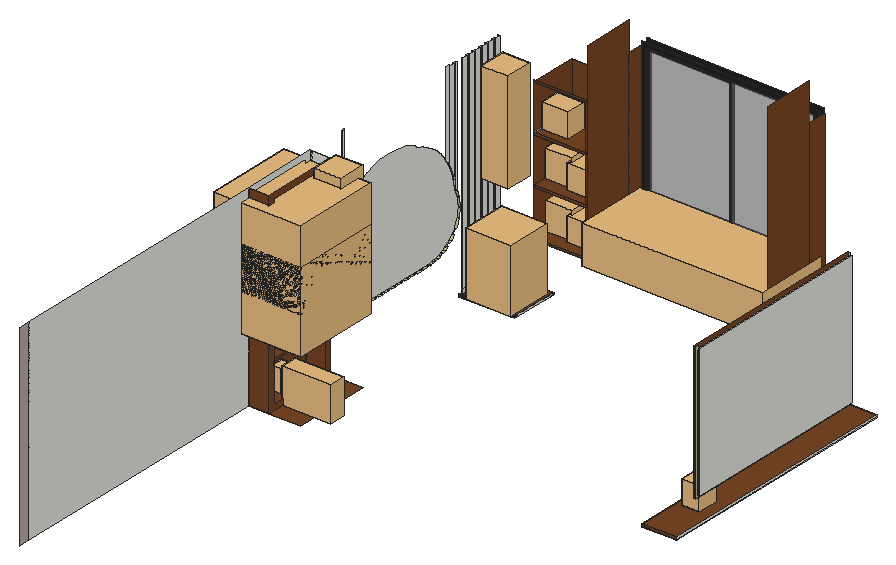
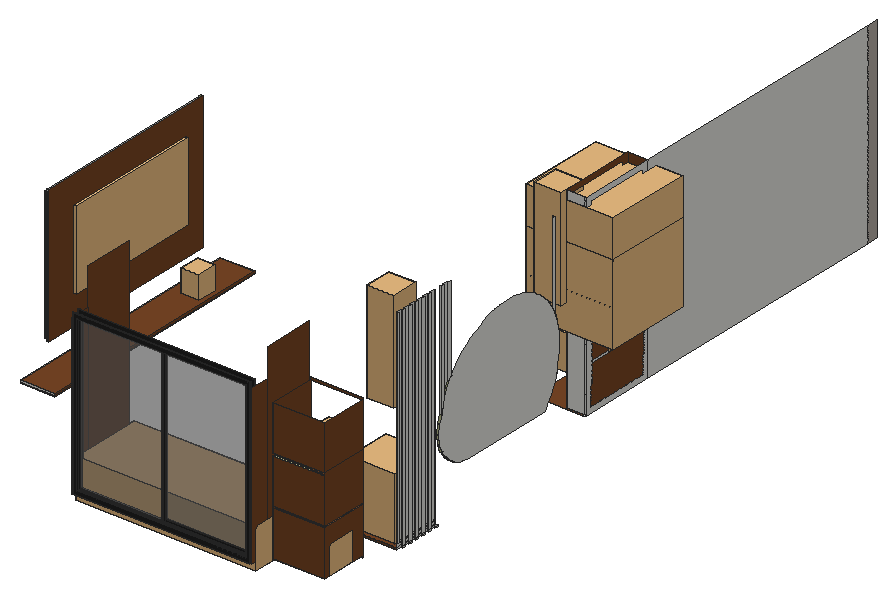
# SketchUp Ruby script. Lengths in inches.
U = 1.inch
M = Sketchup.active_model
def pt(a) = Geom::Point3d.new(a.map { |v| v * U })
def face(e, loops, mat)
  f = e.add_face(loops[0].map { |a| pt(a) })
  loops[1..].each { |l| e.add_face(l.map { |a| pt(a) }).erase! }
  f.material = f.back_material = mat if mat
  f
end
# faces: each face lists its corners as indices into pts; further lists are holes
def faces(e, pts, list, mat = nil) = list.each { |f| face(e, (f[0].is_a?(Array) ? f : [f]).map { |l| l.map { |i| pts[i] } }, mat) }
# xy, xz, yz: faces in a plane at the given z, y or x. An outline is a flat list of corners, or four numbers for a rectangle; further outlines are holes
def ring(l) = l.size == 4 ? [[l[0], l[1]], [l[2], l[1]], [l[2], l[3]], [l[0], l[3]]] : l.each_slice(2).to_a
def flat(e, list, mat, &to3) = list.each { |f| face(e, (f[0].is_a?(Array) ? f : [f]).map { |l| ring(l).map { |u, v| to3.(u, v) } }, mat) }
def xy(e, z, list, mat = nil) = flat(e, list, mat) { |x, y| [x, y, z] }
def xz(e, y, list, mat = nil) = flat(e, list, mat) { |x, z| [x, y, z] }
def yz(e, x, list, mat = nil) = flat(e, list, mat) { |y, z| [x, y, z] }
def lines(e, pts, list) = list.each { |a, b| e.add_line(pt(pts[a]), pt(pts[b])) }
# prism: a flat outline (further loops are holes) pulled along v
def prism(e, loops, v, mat = nil)
  f = face(e, loops, mat); d = Geom::Vector3d.new(v.map { |x| x * U })
  f.pushpull(f.normal.samedirection?(d) ? d.length : -d.length)
end
def box(e, o, s, mat = nil) = prism(e, [[o, [o[0] + s[0], o[1], o[2]], [o[0] + s[0], o[1] + s[1], o[2]], [o[0], o[1] + s[1], o[2]]]], [0, 0, s[2]], mat)
def at(x, y, z, deg = 0) = Geom::Transformation.translation(pt([x, y, z])) * Geom::Transformation.rotation(ORIGIN, Z_AXIS, deg.degrees)
def axes(o, x, y, z) = Geom::Transformation.new([*x, 0, *y, 0, *z, 0, *pt(o).to_a, 1])
def part(name) = M.definitions.add(name)
# library, detail: a bought-in or finely detailed component or shape, given as its bounding box
def library(name, o, s) = part(name).tap { |d| box(d.entities, o, s) }
def detail(e, o, s) = box(e.add_group.entities, o, s)
def put(e, d, t, mat = nil) = e.add_instance(d, t).tap { |i| i.material = mat if mat }
def group(e, t, mat = nil) = e.add_group.tap { |g| g.transformation = t; g.material = mat if mat }.entities
root = M.entities
M.materials.add("Emissive").color = [188, 193, 143]
M.materials.add("Tiles L01 200cm").color = [180, 171, 163]
M.materials.add("[0127_Magenta]").color = [213, 211, 206]
M.materials.add("[0136_Charcoal]").color = [35, 35, 35]
M.materials.add("[Color_006]").color = [86, 86, 86]
M.materials.add("[Translucent Glass Gray]").color = [117, 117, 117]
M.materials["[Translucent Glass Gray]"].alpha = 0.39
M.materials.add("[Translucent_Glass_Gray]").color = [128, 128, 128]
M.materials["[Translucent_Glass_Gray]"].alpha = 0.5
M.materials.add("[Wood Cherry Original]").color = [152, 86, 42]
M.materials.add("[Wood Veneer 01]").color = [120, 70, 37]
c1 = library("Group3\#2",[-226.43,63.68,0],[21.09,21.08,29.58])
c2 = library("Single bed",[-6.74,-2.89,0],[80.16,42.17,34.63])
c3 = library("Vase 005",[-3.71,-4.3,0.02],[8.35,9.45,10.71])
c4 = library("Group2\#1",[-226.96,63.15,0],[23.29,23.68,24.31])
c5 = library("Group3\#1",[-239.85,50.56,0],[44.98,46.36,46.21])
c6 = library("Plant 260 021",[-8.52,-3.8,0.02],[22.57,7.61,16.42])
c7 = part("Window")
box(c7.entities,[0,0,0],[39.75,0.5,77],"[Translucent Glass Gray]")
c8 = part("Slider2")
put(c8.entities,c7,at(1.25,1,1.25),"[Translucent Glass Gray]")
c9 = part("Slider")
prism(c9.entities,[[[0,0,0],[42.25,0,0],[42.25,0,79.5],[0,0,79.5]],[[41,0,1.25],[1.25,0,1.25],[1.25,0,78.25],[41,0,78.25]]],[0,1.5,0],"[0136_Charcoal]")
put(c9.entities,c7,at(1.25,1,1.25),"[Translucent_Glass_Gray]")
c10 = part("Frame\#1")
xy(c10.entities,0,[[0,0,88,0.25],[0,6.25,88,6.5]],"[0136_Charcoal]")
xy(c10.entities,1.25,[[-1,6.25,0,9.5],[88,6.25,89,9.5],[0,6.5,88,9.5]],"[0136_Charcoal]")
xy(c10.entities,2,[[2,0.25,86,6.25]],"[0136_Charcoal]")
xy(c10.entities,2.25,[[2.25,0,85.75,1.25],[2.25,2,85.75,5],[2.25,5.75,85.75,6.5],[88,6.25,89,6.25,88,6.5]],"[0136_Charcoal]")
xy(c10.entities,2.75,[[2.75,1.25,85.25,2],[2.75,5,85.25,5.75]],"[0136_Charcoal]")
xy(c10.entities,81.25,[[2.75,1.25,85.25,2],[2.75,5,85.25,5.75]],"[0136_Charcoal]")
xy(c10.entities,81.75,[[2.25,0,85.75,1.25],[2.25,2,85.75,5],[2.25,5.75,85.75,6.5]],"[0136_Charcoal]")
xy(c10.entities,82,[[2,0.25,86,6.25]],"[0136_Charcoal]")
xy(c10.entities,84,[[0,0,88,0.25],[0,6.25,88,6.5]],"[0136_Charcoal]")
xz(c10.entities,0,[[[0,0,88,84],[2.25,2.25,85.75,81.75]]],"[0136_Charcoal]")
xz(c10.entities,0.25,[[[0,0,88,84],[2,2,86,82]]],"[0136_Charcoal]")
xz(c10.entities,1.25,[[[2.25,2.25,85.75,81.75],[2.75,2.75,85.25,81.25]]],"[0136_Charcoal]")
xz(c10.entities,2,[[[2.25,2.25,85.75,81.75],[2.75,2.75,85.25,81.25]]],"[0136_Charcoal]")
xz(c10.entities,5,[[[2.25,2.25,85.75,81.75],[2.75,2.75,85.25,81.25]]],"[0136_Charcoal]")
xz(c10.entities,5.75,[[[2.25,2.25,85.75,81.75],[2.75,2.75,85.25,81.25]]],"[0136_Charcoal]")
xz(c10.entities,6.25,[[[0,0,88,0,88,1.25,89,1.25,89,2.25,88,2.25,88,84,0,84,0,2.25,-1,2.25,-1,1.25,0,1.25],[2,2,86,82]]],"[0136_Charcoal]")
xz(c10.entities,6.5,[[0,0,88,1.25],[0,2.25,0,84,88,84,88,2.25,85.75,2.25,85.75,81.75,2.25,81.75,2.25,2.25]],"[0136_Charcoal]")
xz(c10.entities,9.5,[[-1,1.25,89,1.75]],"[0136_Charcoal]")
yz(c10.entities,-1,[[6.25,1.25,6.25,2.25,9.5,1.75,9.5,1.25]],"[0136_Charcoal]")
yz(c10.entities,0,[[0,0,0.25,84],[6.25,0,6.5,1.25],[6.25,2.25,6.5,84]],"[0136_Charcoal]")
yz(c10.entities,2,[[0.25,2,6.25,82]],"[0136_Charcoal]")
yz(c10.entities,2.25,[[0,2.25,1.25,81.75],[2,2.25,5,81.75],[5.75,2.25,6.5,81.75]],"[0136_Charcoal]")
yz(c10.entities,2.75,[[1.25,2.75,2,81.25],[5,2.75,5.75,81.25]],"[0136_Charcoal]")
yz(c10.entities,85.25,[[1.25,2.75,2,81.25],[5,2.75,5.75,81.25]],"[0136_Charcoal]")
yz(c10.entities,85.75,[[0,2.25,1.25,81.75],[2,2.25,5,81.75],[5.75,2.25,6.5,81.75]],"[0136_Charcoal]")
yz(c10.entities,86,[[0.25,2,6.25,82]],"[0136_Charcoal]")
yz(c10.entities,88,[[0,0,0.25,84],[6.25,0,6.5,1.25],[6.25,2.25,6.5,84]],"[0136_Charcoal]")
yz(c10.entities,89,[[6.25,1.25,9.5,1.25,9.5,1.75,6.25,2.25]],"[0136_Charcoal]")
p = [[89,6.25,2.25],[89,9.5,1.75],[88,6.5,2.25],[-1,6.25,2.25],[0,6.25,2.25],[-1,9.5,1.75],
  [0,6.5,2.25],[2.25,6.5,2.25],[85.75,6.5,2.25]]
faces(c10.entities,p,[[0,1,2],[3,4,5],[6,5,4],[6,7,8,2,1,5]],"[0136_Charcoal]")
put(c10.entities,c8,axes([1.48,-2.48,1.48],[1.01887,0,0],[0,5.47515,0],[0,0,1.01974]))
put(c10.entities,c9,at(43.5,3.5,2.25),"[Color_006]")
c11 = part("Sliding window \#1")
put(c11.entities,c10,at(-89,-9.5,-1.25),"[Color_006]")
c12 = part("Component")
put(c12.entities,c11,axes([-172.29,84.49,30.25],[-0.94043,0,0],[0,-0.48475,0],[0,0,0.90164]),"[0127_Magenta]")
c13 = part("Sliding window")
put(c13.entities,c12,at(-90.18,103.6875,0))
c14 = part("חלונות")
put(c14.entities,c13,at(48.77,-72.61,0))
c15 = library("Interior Props 221 010",[-4.44,-3.51,-0.03],[8.89,7.03,15.76])
c16 = library("Books 193 006",[-5.22,-3.55,0],[10.44,7.83,2.69])
c17 = library("Flat screen television",[0,1.41,1.14],[35.92,0.28,20.21])
c18 = library("Potted trailing plant",[-13.52,-13.75,-7.41],[40.56,40.5625,37.31])
c19 = library("Books 155 025",[-5.0625,-5.83,0.01],[10.11,11.66,8.59])
c20 = library("Books 297 001 004",[-3.55,-2.96,-0.03],[7.44,5.56,6.72])
c21 = library("Pendant 16-40",[-13.91,-13.91,-52.32],[27.82,27.82,52.32])
xy(root,20.75,[[9,255.72,9,256.96,9.8125,256.96,9.8125,259.39,9,259.39,9,260.76,9.8125,260.76,9.8125,263.18,9,263.18,9,264.55,9.8125,264.55,9.8125,266.97,9,266.97,9,268.34,9.8125,268.34,9.8125,270.77,9,270.77,9,272.13,9.8125,272.13,9.8125,274.56,9,274.56,9,275.92,9.8125,275.92,9.8125,278.35,35,278.35,35,255.72]])
xy(root,21.5625,[[9,255.72,9,256.96,9.8125,256.96,9.8125,259.39,9,259.39,9,260.76,9.8125,260.76,9.8125,263.18,9,263.18,9,264.55,9.8125,264.55,9.8125,266.97,9,266.97,9,268.34,9.8125,268.34,9.8125,270.77,9,270.77,9,272.13,9.8125,272.13,9.8125,274.56,9,274.56,9,275.92,9.8125,275.92,9.8125,278.35,35,278.35,35,255.72]])
xy(root,21.61,[[9,255.72,35,255.72,35,278.35,9.8125,278.35,9.8125,275.92,9,275.92,9,274.56,9.8125,274.56,9.8125,272.13,9,272.13,9,270.77,9.8125,270.77,9.8125,268.34,9,268.34,9,266.97,9.8125,266.97,9.8125,264.55,9,264.55,9,263.18,9.8125,263.18,9.8125,260.76,9,260.76,9,259.39,9.8125,259.39,9.8125,256.96,9,256.96]],"[Wood Veneer 01]")
xy(root,23.75,[[9,256.96,9.8125,259.39],[9,260.76,9.8125,263.18],[9,264.55,9.8125,266.97],[9,268.34,9.8125,270.77],[9,272.13,9.8125,274.56],
  [9,275.92,9.8125,278.35]])
xy(root,25.25,[[35,298.1875,119,322.1875]])
xy(root,25.375,[[173,157.25,173,180.55,185,180.55,185,227.15,173,227.15,173,273.75,189,273.75,189,157.25],[173,180.55,185,227.15]])
xy(root,25.625,[[173,157.25,189,273.75]])
xy(root,26.625,[[173,157.25,189,273.75]],"[Wood Veneer 01]")
xy(root,27,[[10.03,298.1875,34,320.1875]],"[Wood Veneer 01]")
xy(root,29,[[9,133.1875,18.5,168.67],[9,168.67,9.9375,169.5625]])
xy(root,29,[[18.5,133.1875,33.125,133.1875,33.125,169.5625,9.9375,169.5625,9.9375,168.67,18.5,168.67]],"[Wood Veneer 01]")
xy(root,29.13,[[35,322.1875,119,331.1875]])
xy(root,31.59,[[9,135.78,18.5,166.08]],"[Wood Veneer 01]")
xy(root,36.9,[[187.125,169.73,188.1875,259.23]],"[Wood Veneer 01]")
xy(root,38.02,[[188.1875,170.86,189,259.23]],"Emissive")
xy(root,41.75,[[8.625,193.62,9.8125,194.93],[8.625,194.93,9,196.3],[8.625,196.3,9.8125,198.72],[8.625,198.72,9,200.09],[8.625,200.09,9.8125,202.52],
  [8.625,202.52,9,203.88],[8.625,203.88,9.8125,206.31],[8.625,206.31,9,207.67],[8.625,207.67,9.8125,210.1],[8.625,210.1,9,211.46],
  [8.625,211.46,9.8125,213.89],[8.625,213.89,9,215.26],[8.625,215.26,9.8125,217.68],[8.625,217.68,9,219.05],[8.625,219.05,9.8125,221.47],
  [8.625,221.47,9,222.84],[8.625,222.84,9.8125,225.27],[8.625,225.27,9,226.63],[8.625,226.63,9.8125,229.06],[8.625,229.06,9,230.42],
  [8.625,230.42,9.8125,232.85],[8.625,232.85,9,234.21],[8.625,234.21,9.8125,236.64],[8.625,236.64,9,238.01],[8.625,238.01,9.8125,238.43]],"Emissive")
xy(root,48,[[10.03,319.1875,34,320.1875]],"Emissive")
xy(root,48,[[10.03,298.1875,34,319.1875]],"[Wood Veneer 01]")
xy(root,49,[[10,298.1875,34,320.1875]],"[Wood Veneer 01]")
xy(root,49.63,[[9,135.74,10,166.04]],"Emissive")
xy(root,49.63,[[10,135.74,18.5,166.04]],"[Wood Cherry Original]")
xy(root,50.5,[[9,135.73,18.5,166.04]],"[Wood Veneer 01]")
xy(root,68,[[9,135.6875,10,165.99]],"Emissive")
xy(root,68,[[10,135.6875,18.5,165.99]],"[Wood Veneer 01]")
xy(root,69,[[9,135.68,18.5,165.99]],"[Wood Veneer 01]")
xy(root,70,[[10.03,319.1875,34,320.1875]],"Emissive")
xy(root,70,[[10.03,298.1875,34,319.1875]],"[Wood Veneer 01]")
xy(root,71,[[10,298.1875,10.03,320.1875]])
xy(root,71,[[10.03,298.1875,34,320.1875]],"[Wood Veneer 01]")
xz(root,133.1875,[[9,29,18.5,120]],"[Wood Veneer 01]")
xz(root,135.68,[[9,66.57,18.5,69]])
xz(root,135.6875,[[9,66.57,18.5,68]])
xz(root,135.74,[[9,48.07,18.5,49.63]])
xz(root,157.25,[[173,25.375,189,25.625],[173,25.625,189,26.625]],"[Wood Veneer 01]")
xz(root,165.99,[[9,68,18.5,69]])
xz(root,166.04,[[9,49.63,18.5,50.5]])
xz(root,168.67,[[9,29,9.9375,120],[9.9375,29,18.5,120]])
xz(root,169.73,[[187.125,36.9,188.1875,100.27]],"[Wood Veneer 01]")
xz(root,170.86,[[188.1875,38.02,189,99.15]],"Emissive")
xz(root,187.35,[[9,78.74,9.9375,120]])
xz(root,249.38,[[9,78.67,9.8125,120]])
xz(root,251.81,[[9,72.82,9.8125,120]])
xz(root,253.17,[[9,66.43,9.8125,120]])
xz(root,255.72,[[9,21.5625,35,21.61]])
xz(root,255.72,[[9,20.75,35,21.5625]],"[Wood Veneer 01]")
xz(root,256.96,[[9,20.75,9.8125,21.5625],[9,21.5625,9.8125,21.61],[9,21.61,9.8125,23.75],[9,23.75,9.8125,120]])
xz(root,259.23,[[187.125,36.9,188.1875,100.27]])
xz(root,259.23,[[188.1875,38.02,189,99.15]],"Emissive")
xz(root,259.39,[[9,20.75,9.8125,21.5625],[9,21.5625,9.8125,21.61],[9,21.61,9.8125,23.75],[9,23.75,9.8125,120]])
xz(root,260.76,[[9,20.75,9.8125,21.5625],[9,21.5625,9.8125,21.61],[9,21.61,9.8125,23.75],[9,23.75,9.8125,120]])
xz(root,263.18,[[9,20.75,9.8125,21.5625],[9,21.5625,9.8125,21.61],[9,21.61,9.8125,23.75],[9,23.75,9.8125,120]])
xz(root,264.55,[[9,20.75,9.8125,21.5625],[9,21.5625,9.8125,21.61],[9,21.61,9.8125,23.75],[9,23.75,9.8125,120]])
xz(root,266.97,[[9,20.75,9.8125,21.5625],[9,21.5625,9.8125,21.61],[9,21.61,9.8125,23.75],[9,23.75,9.8125,120]])
xz(root,268.34,[[9,20.75,9.8125,21.5625],[9,21.5625,9.8125,21.61],[9,21.61,9.8125,23.75],[9,23.75,9.8125,120]])
xz(root,270.77,[[9,20.75,9.8125,21.5625],[9,21.5625,9.8125,21.61],[9,21.61,9.8125,23.75],[9,23.75,9.8125,120]])
xz(root,272.13,[[9,20.75,9.8125,21.5625],[9,21.5625,9.8125,21.61],[9,21.61,9.8125,23.75],[9,23.75,9.8125,120]])
xz(root,273.75,[[173,25.375,189,25.625],[173,25.625,189,26.625]])
xz(root,274.56,[[9,20.75,9.8125,21.5625],[9,21.5625,9.8125,21.61],[9,21.61,9.8125,23.75],[9,23.75,9.8125,120]])
xz(root,275.92,[[9,20.75,9.8125,21.5625],[9,21.5625,9.8125,21.61],[9,21.61,9.8125,23.75],[9,23.75,9.8125,120]])
xz(root,278.35,[[9,23.75,9.8125,120]])
xz(root,278.35,[[9.8125,20.75,35,21.5625],[9.8125,21.5625,35,21.61]],"[Wood Veneer 01]")
xz(root,298.1875,[[34,26,34.03,48],[34,70,34.03,92]])
xz(root,298.1875,[[10.03,26,34,27],[10,27,10.03,27,10.03,48,34,48,34,49,10,49],[10.03,70,34,71],[10,71,10.03,71,10.03,92,34,92,34,93,10,93]],"[Wood Veneer 01]")
xz(root,320.1875,[[10.03,27,34,48],[10,49,34,49,34,70,10.03,70,10.03,71,10,71],[10.03,71,34,92]],"[Wood Veneer 01]")
xz(root,322.1875,[[35,25.25,119,29.13]])
yz(root,8.625,[[193.62,41.75,238.43,41.75,240.43,42.02,241.8,42.2,242.78,42.32,244.22,42.92,245.59,43.49,246.82,44,248.02,44.92,249.38,45.96,250.3,46.67,251.81,48.63,252.97,50.14,253.17,50.64,254.64,54.19,255.21,58.53,254.64,62.875,253.17,66.43,252.97,66.92,252.5,70.14,251.81,72.82,251.6875,73.28,250.55,76.33,249.1,79.23,248.02,80.92,247.35,81.97,245.59,84.16,245.31,84.5,244.22,85.6,243.03,86.81,241.8,87.8,240.51,88.85,240.43,88.9,238.01,90.48,237.78,90.625,236.64,91.21,234.89,92.1,234.21,92.35,232.85,92.875,231.85,93.26,231.11,93.9,230.42,94.42,230.32,94.49,229.5,95.03,229.06,95.27,228.63,95.5,227.74,95.91,226.82,96.25,226.63,96.31,225.87,96.53,225.27,96.66,224.91,96.74,223.9375,96.88,222.96,96.95,222.84,96.98,222.48,97.0625,222,97.16,221.53,97.26,221.05,97.34,220.5625,97.41,220.08,97.47,219.6,97.52,219.11,97.5625,219.05,97.57,218.625,97.59,218.14,97.61,217.68,97.62,217.16,97.62,216.61,97.7,215.26,97.76,213.89,97.82,213.63,97.83,211.46,97.69,210.66,97.64,210.1,97.54,207.73,97.125,207.67,97.11,206.31,96.72,204.87,96.3,203.88,95.9,202.52,95.34,202.11,95.18,200.09,94.09,199.49,93.76,198.72,93.24,197.04,92.07,196.3,91.4375,194.93,90.26,194.78,90.13,192.75,87.96,192.51,87.65,191.14,85.88,191.14,85.875,189.71,83.67,188.71,81.82,188.46,81.35,187.41,78.93,187.35,78.74,186.57,76.4375,185.9375,73.88,185.51,71.29,185.31,68.66,185.32,66.03,185.55,63.41,186,60.8125,186.66,58.26,186.83,55.63,187.33,53.04,187.35,52.97,188.15,50.54,188.71,49.35,189.28,48.16,190.71,45.9375,191.14,45.43,192.41,43.92,192.51,43.75]])
yz(root,9,[[255.72,20.75,256.96,21.5625],[259.39,20.75,260.76,21.5625],[263.18,20.75,264.55,21.5625],[266.97,20.75,268.34,21.5625],[270.77,20.75,272.13,21.5625],
  [274.56,20.75,275.92,21.5625],[255.72,21.5625,256.96,21.61],[259.39,21.5625,260.76,21.61],[263.18,21.5625,264.55,21.61],[266.97,21.5625,268.34,21.61],
  [270.77,21.5625,272.13,21.61],[274.56,21.5625,275.92,21.61],[259.39,21.61,260.76,120],[263.18,21.61,264.55,120],[266.97,21.61,268.34,120],
  [270.77,21.61,272.13,120],[274.56,21.61,275.92,120],[5.08,29,133.1875,120],[[133.1875,29,168.67,120],[135.78,31.59,166.08,31.59,166.04,50.5,165.99,69,165.95,85.69,165.91,100.13,165.91,102.57,166.08,117.41,135.78,117.41,135.6,102.57,135.6,100.13,135.64,85.69,135.6,85.69,135.6,83.25,135.65,83.25,135.68,69,135.68,66.57,135.6875,66.57,135.73,50.5,135.74,48.07],[135.6875,66.57,135.6875,68,165.99,68,165.99,69,135.68,69],[135.65,83.25,135.65,84.82,165.95,84.82,165.95,85.69,135.64,85.69]],[135.74,48.07,135.73,50.5,166.04,50.5,166.04,49.63,135.74,49.63],
  [253.17,66.43,253.17,120,251.81,120,251.81,72.82,252.5,70.14,252.97,66.92],[135.68,66.57,135.68,69,135.6875,66.57],[135.6875,66.57,135.68,69,165.99,69,165.99,68,135.6875,68],[249.38,78.67,249.38,120,248.02,120,248.02,80.92,249.1,79.23],[187.35,78.74,187.41,78.93,188.46,81.35,188.71,81.82,188.71,120,187.35,120]])
yz(root,9,[[0,29,5.08,120]],"Tiles L01 200cm")
yz(root,9,[[135.78,31.59,166.08,31.59,166.04,50.5,165.99,69,165.95,85.69,165.91,100.13,165.91,101.13,135.6,101.13,135.6,100.13,135.64,85.69,165.95,85.69,165.95,84.82,135.65,84.82,135.65,83.25,135.68,69,165.99,69,165.99,68,135.6875,68,135.6875,66.57,135.73,50.5,166.04,50.5,166.04,49.63,135.74,49.63,135.74,48.07]],"[Wood Veneer 01]")
yz(root,9.8125,[[256.96,20.75,259.39,21.5625],[260.76,20.75,263.18,21.5625],[264.55,20.75,266.97,21.5625],[268.34,20.75,270.77,21.5625],[272.13,20.75,274.56,21.5625],
  [275.92,20.75,278.35,21.5625],[256.96,21.5625,259.39,21.61],[260.76,21.5625,263.18,21.61],[264.55,21.5625,266.97,21.61],[268.34,21.5625,270.77,21.61],
  [272.13,21.5625,274.56,21.61],[275.92,21.5625,278.35,21.61],[256.96,21.61,259.39,23.75],[260.76,21.61,263.18,23.75],[264.55,21.61,266.97,23.75],
  [268.34,21.61,270.77,23.75],[272.13,21.61,274.56,23.75],[275.92,21.61,278.35,23.75],[256.96,23.75,259.39,120],[260.76,23.75,263.18,120],
  [264.55,23.75,266.97,120],[268.34,23.75,270.77,120],[272.13,23.75,274.56,120],[275.92,23.75,278.35,120],[251.81,72.82,251.81,120,249.38,120,249.38,78.67,250.55,76.33,251.6875,73.28]])
yz(root,10,[[298.1875,49,320.1875,71]],"[Wood Veneer 01]")
yz(root,10.03,[[298.1875,70,320.1875,71]])
yz(root,10.03,[[298.1875,27,320.1875,48],[298.1875,71,320.1875,92]],"[Wood Veneer 01]")
yz(root,18.5,[[135.68,66.57,135.6875,66.57,135.68,69]])
yz(root,18.5,[[[133.1875,29,168.67,120],[135.78,31.59,135.74,48.07,135.73,50.5,135.6875,66.57,135.68,69,135.65,83.25,135.6,83.25,135.6,85.69,135.64,85.69,135.6,100.13,135.6,102.57,135.78,117.41,166.08,117.41,165.91,102.57,165.91,100.13,165.95,85.69,165.99,69,166.04,50.5,166.08,31.59],[135.65,83.25,135.64,85.69,165.95,85.69,165.95,84.82,135.65,84.82]],[135.74,48.07,135.74,49.63,166.04,49.63,166.04,50.5,135.73,50.5],[135.6875,66.57,135.6875,68,165.99,68,165.99,69,135.68,69]],"[Wood Veneer 01]")
yz(root,34,[[298.1875,27,320.1875,48],[298.1875,49,320.1875,70],[298.1875,71,320.1875,92]],"[Wood Veneer 01]")
yz(root,35,[[256.86,20.75,277.21,21.5625]])
yz(root,35,[[255.72,20.75,256.86,21.5625],[256.86,20.75,277.21,21.5625],[277.21,20.75,278.35,21.5625],[255.72,21.5625,256.86,21.61],[256.86,21.5625,277.21,21.61],
  [277.21,21.5625,278.35,21.61],[298.1875,25.25,322.1875,116],[322.1875,29.13,331.1875,102.58]],"[Wood Veneer 01]")
yz(root,119,[[298.1875,25.25,322.1875,120],[322.1875,29.13,331.1875,102.58]],"[Wood Veneer 01]")
yz(root,173,[[157.25,25.375,273.75,25.625],[157.25,25.625,273.75,26.625]],"[Wood Veneer 01]")
yz(root,187.125,[[169.73,36.9,259.23,100.27]],"[Wood Veneer 01]")
yz(root,188.1875,[[170.86,38.02,259.23,99.15]])
yz(root,188.1875,[[169.73,36.9,170.86,100.27],[170.86,36.9,259.23,38.02]],"Emissive")
yz(root,189,[[157.25,25.375,273.75,25.625],[157.25,25.625,273.75,26.625],[170.86,38.02,259.23,99.15]])
p = [[9,135.78,31.59],[9,135.74,48.07],[18.5,135.74,48.07],[18.5,135.78,31.59],[9,166.04,50.5],[9,166.08,31.59],
  [18.5,166.08,31.59],[18.5,166.04,50.5],[8.625,192.51,43.75],[9,192.51,43.75],[9.8125,192.51,43.75],[9.8125,193.62,41.75],
  [8.625,193.62,41.75],[8.625,238.43,41.75],[9.8125,238.43,41.75],[9.8125,240.43,42.02],[9,240.43,42.02],[8.625,240.43,42.02],
  [9,241.8,42.2],[8.625,241.8,42.2],[9.8125,241.8,42.2],[9.8125,242.78,42.32],[8.625,242.78,42.32],[9.8125,244.22,42.92],
  [9,244.22,42.92],[8.625,244.22,42.92],[9,245.59,43.49],[8.625,245.59,43.49],[9.8125,245.59,43.49],[9.8125,246.82,44],
  [8.625,246.82,44],[9,192.41,43.92],[8.625,192.41,43.92],[9,191.14,45.43],[8.625,191.14,45.43],[9.8125,248.02,44.92],
  [9,248.02,44.92],[8.625,248.02,44.92],[9,249.38,45.96],[8.625,249.38,45.96],[8.625,190.71,45.9375],[9.8125,190.71,45.9375],
  [9.8125,191.14,45.43],[8.625,189.28,48.16],[9.8125,189.28,48.16],[9.8125,249.38,45.96],[9.8125,250.3,46.67],[8.625,250.3,46.67],
  [9.8125,251.81,48.63],[9,251.81,48.63],[8.625,251.81,48.63],[9,135.73,50.5],[18.5,135.73,50.5],[8.625,188.71,49.35],
  [9,188.71,49.35],[9.8125,188.71,49.35],[9,252.97,50.14],[8.625,252.97,50.14],[9,188.15,50.54],[8.625,188.15,50.54],
  [9,253.17,50.64],[8.625,253.17,50.64],[9,135.6875,66.57],[18.5,135.6875,66.57],[9,165.99,69],[18.5,165.99,69],
  [9,187.35,52.97],[8.625,187.35,52.97],[9.8125,253.17,50.64],[9.8125,254.64,54.19],[8.625,254.64,54.19],[8.625,186.83,55.63],
  [9.9375,186.83,55.63],[9.9375,187.33,53.04],[8.625,187.33,53.04],[9.9375,187.35,52.97],[9.8125,255.21,58.53],[8.625,255.21,58.53],
  [8.625,186.66,58.26],[9.9375,186.66,58.26],[8.625,186,60.8125],[9.9375,186,60.8125],[9.8125,254.64,62.875],[8.625,254.64,62.875],
  [8.625,185.55,63.41],[9.9375,185.55,63.41],[9.8125,253.17,66.43],[9,253.17,66.43],[8.625,253.17,66.43],[8.625,185.32,66.03],
  [9.9375,185.32,66.03],[8.625,185.31,68.66],[9.9375,185.31,68.66],[9,252.97,66.92],[8.625,252.97,66.92],[9,135.68,69],
  [18.5,135.68,69],[9,252.5,70.14],[8.625,252.5,70.14],[8.625,185.51,71.29],[9.9375,185.51,71.29],[9,135.65,83.25],
  [18.5,135.65,83.25],[9,165.95,85.69],[18.5,165.95,85.69],[9,251.81,72.82],[8.625,251.81,72.82],[8.625,185.9375,73.88],
  [9.9375,185.9375,73.88],[9.8125,251.81,72.82],[9.8125,251.6875,73.28],[8.625,251.6875,73.28],[9.8125,250.55,76.33],[8.625,250.55,76.33],
  [8.625,186.57,76.4375],[9.9375,186.57,76.4375],[9.8125,249.38,78.67],[9,249.38,78.67],[8.625,249.38,78.67],[8.625,187.35,78.74],
  [9,187.35,78.74],[9.9375,187.35,78.74],[9,187.41,78.93],[8.625,187.41,78.93],[9,249.1,79.23],[8.625,249.1,79.23],
  [9,188.46,81.35],[8.625,188.46,81.35],[9,248.02,80.92],[8.625,248.02,80.92]]
faces(root,p,[[0,1,2,3],[1,51,52,2],[51,62,63,52],[62,95,96,63],[95,101,102,96]])
faces(root,p,[[4,5,6,7],[64,4,7,65],[103,64,65,104]],"[Wood Veneer 01]")
faces(root,p,[[8,9,10,11,12],[13,14,15,16,17],[16,18,19,17],[19,18,20,21,22],[22,21,23,24,25],[24,26,27,25],[27,26,28,29,30],[31,9,8,32],
  [33,31,32,34],[30,29,35,36,37],[36,38,39,37],[40,41,42,33,34],[43,44,41,40],[39,38,45,46,47],[47,46,48,49,50],[53,54,55,44,43],
  [49,56,57,50],[58,54,53,59],[56,60,61,57],[66,58,59,67],[61,60,68,69,70],[71,72,73,74],[74,73,75,66,67],[70,69,76,77],
  [78,79,72,71],[80,81,79,78],[77,76,82,83],[84,85,81,80],[83,82,86,87,88],[89,90,85,84],[91,92,90,89],[87,93,94,88],
  [93,97,98,94],[99,100,92,91],[97,105,106,98],[107,108,100,99],[106,105,109,110,111],[111,110,112,113],[114,115,108,107],[113,112,116,117,118],
  [119,120,121,115,114],[122,120,119,123],[117,124,125,118],[126,122,123,127],[124,128,129,125]],"Emissive")
put(root,c1,at(238.88,191.44,21.19))
put(root,c2,axes([111.94,326.55,25.25],[-1.048,0,0],[0,-0.80763,0],[0,0,0.53]))
put(root,c3,at(178.9,181.7,26.625))
put(root,c4,axes([130.3125,271.08,27],[0.53,0,0],[0,0.53,0],[0,0,0.53]))
put(root,c5,axes([78.95,290.76,27],[0.24,0,0],[0,0.24,0],[0,0,0.24]))
put(root,c6,at(26.84,144.68,29))
put(root,c14,at(248.7,211.14,0))
put(root,c15,axes([13.46,146.52,31.58],[0,0.66,0],[-0.66,0,0],[0,0,0.66]))
put(root,c4,axes([130.3125,271.08,49],[0.53,0,0],[0,0.53,0],[0,0,0.53]))
put(root,c5,axes([78.95,290.76,49],[0.24,0,0],[0,0.24,0],[0,0,0.24]))
put(root,c16,axes([12.68,149.64,50.5],[0,-1.3338,0],[1.14,0,0],[0,0,1.14]))
put(root,c17,axes([177.96,245.27,49.33],[0,-1.8125,0],[5.4375,0,0],[0,0,1.8125]))
put(root,c18,at(23.28,142.14,68.5625,90))
put(root,c19,axes([13.93,147.97,69],[1.09,0,0],[0,1.09,0],[0,0,1.09]))
put(root,c20,axes([16.31,306.875,71.05],[1.66,0,0],[0,1.66,0],[0,0,1.66]))
put(root,c21,axes([24.67,263.08,120],[0.45,0,0],[0,0.45,0],[0,0,0.9]))
put(root,c21,axes([24.76,165.65,120],[0.45,0,0],[0,0.45,0],[0,0,0.9]))
put(root,c18,at(23.28,142.14,86.0625,90))
